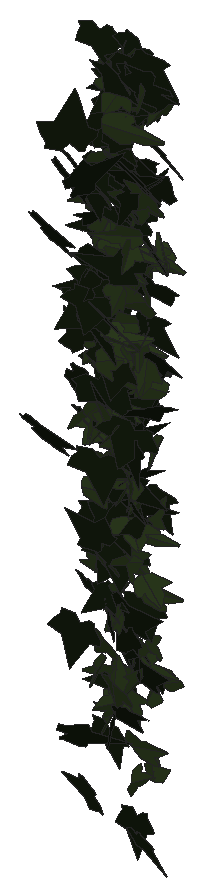
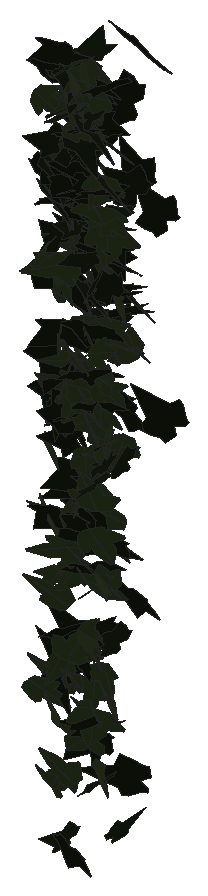
# SketchUp Ruby script. Lengths in millimetres.
U = 1.mm
M = Sketchup.active_model
def pt(a) = Geom::Point3d.new(a.map { |v| v * U })
def face(e, loops, mat)
  f = e.add_face(loops[0].map { |a| pt(a) })
  loops[1..].each { |l| e.add_face(l.map { |a| pt(a) }).erase! }
  f.material = f.back_material = mat if mat
  f
end
# faces: each face lists its corners as indices into pts; further lists are holes
def faces(e, pts, list, mat = nil) = list.each { |f| face(e, (f[0].is_a?(Array) ? f : [f]).map { |l| l.map { |i| pts[i] } }, mat) }
# xy, xz, yz: faces in a plane at the given z, y or x. An outline is a flat list of corners, or four numbers for a rectangle; further outlines are holes
def ring(l) = l.size == 4 ? [[l[0], l[1]], [l[2], l[1]], [l[2], l[3]], [l[0], l[3]]] : l.each_slice(2).to_a
def flat(e, list, mat, &to3) = list.each { |f| face(e, (f[0].is_a?(Array) ? f : [f]).map { |l| ring(l).map { |u, v| to3.(u, v) } }, mat) }
def xy(e, z, list, mat = nil) = flat(e, list, mat) { |x, y| [x, y, z] }
def xz(e, y, list, mat = nil) = flat(e, list, mat) { |x, z| [x, y, z] }
def yz(e, x, list, mat = nil) = flat(e, list, mat) { |y, z| [x, y, z] }
def lines(e, pts, list) = list.each { |a, b| e.add_line(pt(pts[a]), pt(pts[b])) }
# prism: a flat outline (further loops are holes) pulled along v
def prism(e, loops, v, mat = nil)
  f = face(e, loops, mat); d = Geom::Vector3d.new(v.map { |x| x * U })
  f.pushpull(f.normal.samedirection?(d) ? d.length : -d.length)
end
def box(e, o, s, mat = nil) = prism(e, [[o, [o[0] + s[0], o[1], o[2]], [o[0] + s[0], o[1] + s[1], o[2]], [o[0], o[1] + s[1], o[2]]]], [0, 0, s[2]], mat)
def at(x, y, z, deg = 0) = Geom::Transformation.translation(pt([x, y, z])) * Geom::Transformation.rotation(ORIGIN, Z_AXIS, deg.degrees)
def axes(o, x, y, z) = Geom::Transformation.new([*x, 0, *y, 0, *z, 0, *pt(o).to_a, 1])
def part(name) = M.definitions.add(name)
# library, detail: a bought-in or finely detailed component or shape, given as its bounding box
def library(name, o, s) = part(name).tap { |d| box(d.entities, o, s) }
def detail(e, o, s) = box(e.add_group.entities, o, s)
def put(e, d, t, mat = nil) = e.add_instance(d, t).tap { |i| i.material = mat if mat }
def group(e, t, mat = nil) = e.add_group.tap { |g| g.transformation = t; g.material = mat if mat }.entities
root = M.entities
M.materials.add("efeu1").color = [18, 25, 13]
M.materials.add("efeu2").color = [43, 57, 29]
c1 = part("ivyleaf_9")
p = [[39.1,54.8,31.7],[34.5,51.8,30.2],[-5.3,25.2,17.3],[-17.9,28.3,20.9],[-21.6,21.7,17],[-20.2,4.3,5.3],
  [-22.9,-0.3,2.5],[-17.1,-4,-0.6],[-2,-2.1,-1.2],[-0.7,-15.4,-10.1],[16.6,-22.3,-16.7],[21.1,-15.1,-12.5],
  [32.7,-10.7,-11],[46.1,-1.8,-6.6],[30.8,11.2,3.8]]
faces(c1.entities,p,[[0,1,2,3,4,5,6,7,8,9,10,11,12,13,14]],"efeu1")
c2 = part("ivyleaf_10")
p = [[0,12.8,-0.8],[-1.5,51.3,-10.9],[-4.9,51,-11.6],[-13.6,26.5,-7.3],[-13.2,15.9,-4.6],[-21.1,19.3,-7.2],
  [-29.5,16.3,-8.3],[-29.2,8.3,-6.2],[-19.7,-9.8,0.5],[-7.6,-13,4],[1,-12.2,5.8],[-0.4,51.1,-11.1],
  [-1.5,51.1,-10.9],[1,-12.4,5.9],[16.9,-12.4,3.5],[35.1,9.1,-5.1],[35,12.9,-6.1],[20.5,16.4,-4.9],
  [15.8,15,-3.8],[15.3,27.6,-7.1],[12.8,31.3,-7.8]]
faces(c2.entities,p,[[0,1,2,3,4,5,6,7,8,9,10],[11,12,0,13,14,15,16,17,18,19,20]],"efeu2")
put(root,c1,axes([2484.9,735.8,1568],[-1.69227,0.67387,-0.10406],[-0.16332,0.05905,1.11567],[1.2874,0.89329,0.00475]))
put(root,c1,axes([2483.9,756.8,1476.8],[0.18465,0.07319,1.16134],[1.50191,0.8523,-0.11964],[-1.62756,0.7948,0.02135]))
put(root,c1,axes([2359.6,808.1,967.1],[1.40617,-0.08875,-0.62221],[1.17808,-0.06371,0.74411],[-0.20734,-0.96384,0.00811]))
put(root,c1,axes([2446.9,808.4,638.2],[-1.43808,0.002,-0.59826],[1.13852,-0.01008,-0.75558],[-0.01488,-0.96372,0.00666]))
put(root,c1,axes([2369,814.9,1335.4],[1.32826,-0.24708,-0.62973],[1.18689,-0.11557,0.73649],[-0.49882,-0.93289,0.07555]))
put(root,c1,axes([2392.2,851.2,1410.2],[-0.15635,-0.25819,0.96773],[0.53476,-0.93793,-0.22639],[1.82966,0.25207,0.14886]))
put(root,c2,axes([2459.1,851.1,1104.8],[0.566,-0.46163,-0.60165],[0.85277,-0.41442,0.53946],[-1.1644,-0.5279,0.10262]))
put(root,c1,axes([2459.1,853.3,1185.9],[0.68758,-0.5464,0.48417],[0.54213,-0.39189,-0.65481],[1.2793,0.45974,0.01727]))
put(root,c2,axes([2516,854.7,1330],[0.21144,0.59983,-0.55383],[-0.20997,-0.54278,-0.60999],[-1.53954,0.15641,0.00713]))
put(root,c1,axes([2517.1,853.1,1286.2],[-0.55429,0.00633,0.77085],[-1.46054,-0.08043,-0.28928],[0.13896,-0.8201,0.03432]))
put(root,c2,axes([2516.4,856.2,1350.7],[0.02984,0.15758,-0.80777],[-1.38592,-0.37377,-0.08705],[-0.72979,0.71626,0.13228]))
put(root,c1,axes([2435.9,859.7,1206.7],[-0.72098,-0.71589,0.04601],[-0.02643,-0.0447,-0.80989],[1.36503,-0.37898,0.00862]))
put(root,c1,axes([2446.5,861.6,915.6],[-0.48339,-0.87749,-0.09441],[0.07234,0.08727,-0.91342],[1.67811,-0.25653,0.01218]))
put(root,c1,axes([2479.8,871.4,1613.7],[-0.83606,-0.37476,0.71593],[0.0898,-0.82538,-0.4031],[1.53532,-0.1558,0.41343]))
put(root,c1,axes([2425.7,874.3,1149.4],[0.21537,-0.82051,0.52307],[0.37692,-0.49615,-0.82113],[1.81316,0.2006,0.10856]))
put(root,c1,axes([2423.3,881.9,1175.4],[-1.04304,-0.56212,0.5967],[-0.62623,-0.50657,-0.77943],[1.429,-0.63229,0.09397]))
put(root,c1,axes([2441.7,866,1263.9],[-0.16971,-0.08834,0.95115],[1.68448,-0.367,0.04889],[0.68391,0.88201,0.11561]))
put(root,c2,axes([2476.4,871.2,1226.7],[1.15926,-0.71971,0.06776],[0.0676,-0.05871,-0.94281],[1.37415,0.61005,-0.01078]))
put(root,c1,axes([2458.8,884.7,1092.2],[-0.36321,-0.88951,0.3733],[-0.07063,-0.37348,-0.90892],[1.83459,-0.19048,0.03891]))
put(root,c2,axes([2512.3,857.3,886],[0.46586,-0.6296,-0.63071],[-0.12077,0.64009,-0.6636],[1.69178,0.21907,0.1263]))
put(root,c1,axes([2498.5,877.7,947.7],[-0.56617,-0.01021,-0.78546],[1.44293,-0.22351,-0.28423],[-0.3912,-0.80962,0.08837]))
put(root,c1,axes([2500.2,874.9,1413.2],[-1.0248,0.23639,-0.57178],[0.98332,-0.24522,-0.58794],[-0.64782,-0.74615,0.01208]))
put(root,c1,axes([2426.6,863.2,1221.4],[-0.90472,0.61769,0.22037],[-0.29716,0.15775,-0.77898],[-1.21228,-0.49965,0.02649]))
put(root,c2,axes([2474,872,1598.9],[1.5296,-0.57535,-0.12169],[-0.18897,0.07036,-0.98841],[1.10316,0.80981,-0.00058]))
put(root,c2,axes([2460.8,886,955.1],[-0.09591,0.01155,-0.83258],[-0.30336,-0.81881,-0.00171],[-1.55541,0.15899,0.05167]))
put(root,c1,axes([2413.1,859.6,1125.8],[-1.12518,0.24381,-0.4919],[-0.86458,0.18867,0.6395],[0.58672,0.74558,-0.00097]))
put(root,c2,axes([2528.3,868.9,1425.2],[-1.31885,0.28336,0.34939],[-0.66883,0.05958,-0.74533],[-0.53448,-0.77377,0.07056]))
put(root,c1,axes([2494.9,887.1,972.8],[-1.09181,-0.65305,-0.05444],[0.06639,0.04182,-0.86924],[1.24544,-0.57473,-0.00139]))
put(root,c1,axes([2367,892.6,1416.7],[0.54315,-0.58014,0.71659],[0.59216,-0.64553,-0.64653],[1.6518,0.42218,-0.00386]))
put(root,c2,axes([2473.7,889,1111.7],[-0.98102,-0.38488,-0.46913],[-0.56714,-0.37564,0.63561],[-1.00603,0.58709,0.09914]))
put(root,c2,axes([2451.3,880.8,1278.5],[0.56832,0.02888,0.8239],[1.55948,0.08607,-0.3],[-0.17272,0.87211,0.00232]))
put(root,c2,axes([2462,881,1521.9],[0.05458,0.00345,-0.99141],[1.85453,-0.18293,0.02755],[-0.34783,-0.97481,-0.00868]))
put(root,c1,axes([2436.7,872.7,758.5],[-0.24148,0.29665,0.76444],[-0.81568,0.63548,-0.31774],[-1.33046,-0.44344,0.05606]))
put(root,c1,axes([2468.9,881.4,1458.6],[1.70609,-0.3728,-0.19959],[-0.33754,0.09323,-0.9707],[0.7306,0.91364,0.01761]))
put(root,c1,axes([2410.1,903.2,1216],[-0.7247,-0.68788,0.31013],[-0.28527,-0.27151,-0.78624],[1.40746,-0.40922,0.00033]))
put(root,c2,axes([2461.6,874.1,1131.4],[0.41055,-0.12873,-0.94919],[1.27533,0.71553,0.05525],[1.30268,-0.65993,0.24506]))
put(root,c2,axes([2460.8,883.8,494],[-1.27268,0.45432,0.25237],[-0.41429,0.12859,-0.80829],[-0.89816,-0.70308,0.01524]))
put(root,c2,axes([2448,888.4,1286.8],[-0.02144,-0.10949,-0.99075],[1.88284,0.11993,-0.0245],[0.23197,-0.98353,0.10731]))
put(root,c2,axes([2504.1,891.7,1592.1],[0.71636,-0.77323,-0.24016],[-0.08204,0.24533,-0.85743],[1.53877,0.37305,0.06609]))
put(root,c2,axes([2495.2,891.7,1393.8],[-1.7657,-0.00435,0.0386],[-0.07344,-0.00217,-0.92776],[0.00844,-0.92856,0.00198]))
put(root,c1,axes([2491.6,905,524.7],[0.03789,-0.07783,0.86073],[0.75048,-0.7653,-0.07832],[1.46364,0.39442,0.01787]))
put(root,c1,axes([2363.8,901.8,1027],[0.26318,-0.14266,-0.76129],[1.4741,0.02489,0.13602],[-0.0011,-0.77334,0.14481]))
put(root,c2,axes([2419.3,898.7,982.5],[-0.75661,0.59175,-0.36069],[0.35139,-0.31035,-0.71267],[-1.27126,-0.43797,0.01768]))
put(root,c1,axes([2388.7,910.9,1370.4],[-0.02988,-0.7081,0.43658],[0.21345,-0.43447,-0.70065],[1.56876,0.04563,0.10365]))
put(root,c2,axes([2477.4,894.2,1110.8],[-0.623,0.73544,-0.06457],[-0.11512,0.04367,0.80413],[1.40035,0.33078,0.03738]))
put(root,c2,axes([2477.1,896.1,874.1],[0.84548,-0.00115,-0.6705],[-1.2603,0.12545,-0.43895],[0.20023,0.79447,0.06834]))
put(root,c2,axes([2495.8,906.5,519.9],[-0.03194,-0.71517,0.4305],[-0.03508,-0.43017,-0.71533],[1.5883,-0.02388,-0.00714]))
put(root,c1,axes([2474.9,892.2,1506.5],[-1.21577,0.56264,0.37307],[-0.55706,0.232,-0.85107],[-1.15779,-0.70244,0.01773]))
put(root,c2,axes([2415.7,905.7,1131.7],[1.16675,-0.31717,0.59025],[1.00601,-0.26275,-0.6902],[0.78375,0.80943,0.00724]))
put(root,c1,axes([2485.1,909.1,1591.8],[-1.79302,-0.33008,0.09395],[-0.16024,-0.04378,-0.99817],[0.6332,-0.94577,0.01342]))
put(root,c2,axes([2429.3,899.2,689.7],[-1.35531,0.22483,-0.27772],[-0.5332,0.03304,0.74513],[0.42209,0.76365,0.04953]))
put(root,c1,axes([2515.8,904.9,1606.6],[-0.02814,-0.04533,-0.99131],[-1.33466,-0.70098,0.04252],[-1.33625,0.7011,-0.02159]))
put(root,c1,axes([2420,895.8,1034.6],[-0.23842,-0.55746,-0.72596],[0.40486,0.69493,-0.57034],[1.69431,-0.2445,0.03413]))
put(root,c1,axes([2393.2,909.2,261],[0.29829,-0.79501,0.05984],[0.00837,0.06185,0.81015],[-1.51732,-0.15595,0.01623]))
put(root,c2,axes([2459.4,898.9,915.3],[-0.59112,-0.84992,-0.15469],[0.09705,0.14606,-0.90489],[1.64127,-0.31474,-0.0022]))
put(root,c1,axes([2489,907.4,220.9],[0.68986,-0.66754,0.13765],[0.11779,-0.12302,-0.75959],[1.29183,0.3677,-0.00425]))
put(root,c2,axes([2455.9,916.3,1324.7],[-0.34755,0.1429,-0.82601],[0.4308,-0.80557,-0.18941],[-1.53615,-0.25825,0.13376]))
put(root,c2,axes([2505.1,906.1,1219.3],[-0.87736,0.62911,0.2138],[0.24356,-0.17128,0.77993],[1.24089,0.47842,-0.00192]))
put(root,c2,axes([2414.7,919.7,954.5],[0.06673,-0.54942,0.77103],[0.31553,-0.75608,-0.54631],[1.77404,0.15514,0.06816]))
put(root,c2,axes([2500.7,900.3,1204.7],[-0.93079,0.03641,0.64444],[-1.22526,0.03067,-0.49031],[-0.0884,-0.80842,0.01042]))
put(root,c2,axes([2463.4,912.3,1148.3],[0.10461,0.09973,-0.81363],[-1.38113,-0.37331,-0.09478],[-0.72552,0.72503,0.06312]))
put(root,c2,axes([2475.2,902.3,789.6],[1.26142,0.41634,0.17648],[0.27626,0.10067,-0.78267],[-0.81508,0.67845,0.00784]))
put(root,c2,axes([2409.9,909.3,510.2],[0.56971,-0.80877,0.14102],[0.08815,-0.13323,-0.86239],[1.55999,0.30289,-0.00277]))
put(root,c2,axes([2457.7,914.3,707.2],[0.50814,-0.50082,-0.66025],[0.71823,-0.54409,0.56532],[-1.40416,-0.45954,0.05023]))
put(root,c1,axes([2473.9,908.8,801.7],[-1.67884,0.19549,-0.12307],[0.22811,-0.02797,-0.90351],[-0.37584,-0.89022,0.00136]))
put(root,c2,axes([2395.9,905.5,826.4],[0.26841,-0.11162,-0.76977],[1.43793,-0.16626,0.16253],[-0.3518,-0.76471,0.07702]))
put(root,c1,axes([2418.1,902.7,1412.7],[-0.11458,-0.71576,-0.66616],[0.21359,0.65795,-0.71709],[1.84865,-0.12038,0.04156]))
put(root,c1,axes([2426.2,916.4,387.2],[0.16512,0.29022,0.86965],[-0.45978,-0.83543,0.3029],[1.68319,-0.25667,-0.00257]))
put(root,c1,axes([2429.8,922.6,1528.4],[0.02318,-0.06148,-0.96523],[0.50432,-0.92816,0.06246],[-1.77032,-0.26521,0.00516]))
put(root,c2,axes([2409.9,908.9,947.8],[1.16959,0.40623,-0.30525],[-0.49104,-0.16322,-0.73665],[-0.83314,0.66648,0.00565]))
put(root,c1,axes([2357.9,896.6,367.3],[0.86201,0.05067,0.6925],[1.30331,0.10406,-0.45551],[-0.21842,0.82089,0.01499]))
put(root,c2,axes([2432,922.4,442.3],[-0.01005,0.14021,0.91001],[0.20894,-0.90344,0.13984],[1.73987,0.1093,-0.01154]))
put(root,c2,axes([2399.1,917.7,958.5],[0.16243,-0.6148,0.53097],[0.32302,-0.50862,-0.61619],[1.51194,0.17471,0.0746]))
put(root,c2,axes([2384.2,898.3,964.1],[-0.34505,-0.7313,-0.51435],[0.42117,0.47178,-0.74879],[1.64864,-0.27358,0.08364]))
put(root,c2,axes([2375.9,892.5,1130],[-0.17168,-0.51212,0.82096],[0.26811,0.80878,0.52001],[-1.82191,0.16728,-0.00083]))
put(root,c1,axes([2457.5,899.5,861.3],[0.01689,-0.15204,-0.78653],[0.52551,0.73896,-0.13973],[1.43121,-0.26954,0.06059]))
put(root,c2,axes([2390.3,910.2,1229],[0.3966,-0.7691,-0.01612],[-0.00058,0.01662,-0.79682],[1.46408,0.20835,0.00405]))
put(root,c1,axes([2422.3,905.9,1498.2],[0.3294,-0.67643,-0.52752],[-0.12616,0.52599,-0.69622],[1.6277,0.17766,0.05279]))
put(root,c1,axes([2439.9,918.8,732.1],[-0.74317,-0.86408,-0.18766],[0.1456,0.17136,-0.94821],[1.67654,-0.39791,-0.00084]))
put(root,c1,axes([2509.7,896.6,1012.8],[0.80838,0.68591,0.09505],[0.09665,0.08035,-0.80678],[-1.31435,0.42777,-0.00087]))
put(root,c2,axes([2490.5,895,330.6],[-0.08441,-0.2532,-0.78851],[0.39787,0.76065,-0.25601],[1.52512,-0.21245,0.02315]))
put(root,c1,axes([2419.1,923.9,581.6],[-0.08461,0.00443,0.82284],[-0.23626,-0.81465,-0.00232],[1.54814,-0.12408,0.04462]))
put(root,c2,axes([2460.7,901.9,987],[0.37576,0.68911,0.3655],[0.20082,0.34997,-0.71682],[-1.47093,0.22382,-0.0045]))
put(root,c2,axes([2507.7,905.2,694.4],[0.58066,0.71883,0.224],[0.1788,0.20346,-0.78087],[-1.42176,0.31916,-0.00672]))
put(root,c2,axes([2463.8,907.2,1298.9],[0.55177,-0.90055,0.27936],[-0.16476,0.26561,0.94607],[-1.78692,-0.30256,-0.00097]))
put(root,c2,axes([2411,922.7,723.4],[0.44251,-0.75546,0.49666],[0.32069,-0.46763,-0.79018],[1.69053,0.28646,0.01989]))
put(root,c1,axes([2491.5,926.1,1300.7],[0.3191,-0.62273,0.60556],[0.29903,-0.58482,-0.6449],[1.62588,0.22978,-0.00024]))
put(root,c2,axes([2492.2,916.5,1079.2],[1.51671,-0.40304,0.19952],[0.32967,-0.09954,-0.89299],[0.78987,0.81547,-0.0104]))
put(root,c1,axes([2476.7,911.5,1637.2],[-0.28975,-0.36617,-0.83759],[1.2348,0.55489,-0.36051],[1.22559,-0.64562,0.1652]))
put(root,c1,axes([2415.7,931.5,706.6],[-0.365,-0.75154,0.58031],[-0.29867,-0.5588,-0.77555],[1.78226,-0.24756,-0.01112]))
put(root,c1,axes([2454.8,920.6,571.7],[-0.59754,0.07614,-0.87026],[1.6259,-0.16647,-0.32277],[-0.3474,-0.91006,-0.01376]))
put(root,c1,axes([2498.4,909.4,1347.5],[-1.08381,0.40005,0.5151],[-0.86384,0.24796,-0.69438],[-0.89136,-0.72673,0.04663]))
put(root,c1,axes([2414.7,928,632.9],[0.1509,-0.18932,-0.73874],[0.40478,-0.70776,0.20421],[-1.39382,-0.22604,-0.02068]))
put(root,c1,axes([2421.2,915,789.8],[-0.83272,-0.4306,-0.66005],[0.86062,0.48113,-0.61363],[1.2284,-0.62898,-0.01753]))
put(root,c2,axes([2446.7,928,1081],[0.32007,0.25385,-0.85963],[-0.98082,-0.68821,-0.30405],[-1.39572,0.54185,0.01654]))
put(root,c1,axes([2486.8,911.9,1424.9],[0.50363,0.55929,-0.58872],[-0.69098,-0.47236,-0.61194],[-1.38238,0.43987,0.0914]))
put(root,c2,axes([2408.3,923.4,1307.7],[-0.08665,-0.77495,0.37342],[0.17963,-0.37618,-0.76918],[1.6273,0.00026,0.10479]))
put(root,c2,axes([2408.3,920.2,1174.6],[-0.84553,-0.33049,0.57072],[-0.85009,-0.35551,-0.55356],[0.92347,-0.62985,0.01298]))
put(root,c2,axes([2508.8,925.1,1039.5],[0.21911,0.14111,0.83023],[-0.97357,-0.65393,0.18208],[1.27319,-0.52432,-0.00365]))
put(root,c1,axes([2419.3,922.5,843],[0.14826,0.00901,-0.93338],[1.77187,-0.06824,0.07704],[-0.12802,-0.93414,-0.01463]))
put(root,c1,axes([2363.7,920.1,946.5],[0.93276,-0.63824,0.10982],[0.10766,-0.095,-0.80461],[1.22784,0.49319,-0.01287]))
put(root,c2,axes([2466,903.3,853.6],[-0.01823,-0.59114,-0.69461],[0.05802,0.69405,-0.59109],[1.73494,-0.02942,0.01247]))
put(root,c1,axes([2446.3,926.9,1396.9],[0.11451,-0.78991,0.12088],[0.03643,-0.11977,-0.79214],[1.52042,0.06236,0.00987]))
put(root,c2,axes([2495,924.8,1252.1],[0.05538,-0.80641,0.29743],[0.0463,-0.2967,-0.80683],[1.63516,0.03571,0.01277]))
put(root,c1,axes([2444.9,925.3,598.6],[-0.05958,0.01978,0.9289],[1.01582,-0.76038,0.03418],[1.44738,0.53447,0.01425]))
put(root,c1,axes([2510,916.2,1235.1],[0.43999,0.32532,-0.72399],[-1.10177,-0.44678,-0.38561],[-1.03345,0.61481,0.10287]))
put(root,c2,axes([2415.7,920.7,1313.4],[1.4361,-0.16498,0.20367],[0.38222,-0.03491,-0.77235],[0.32054,0.78079,0.00851]))
put(root,c1,axes([2448.2,926.5,1343.7],[0.56205,-0.75516,0.18422],[0.19421,-0.1577,-0.81003],[1.46657,0.31029,0.03666]))
put(root,c1,axes([2413,914.8,1327.2],[0.38222,0.62114,-0.45863],[-0.44727,-0.40223,-0.64766],[-1.39976,0.29813,0.08172]))
put(root,c2,axes([2416,910.7,550],[-1.05159,0.30245,0.48443],[-0.8221,0.2196,-0.62979],[-0.71099,-0.70125,0.01171]))
put(root,c2,axes([2464.7,911.1,719.3],[-0.8336,-0.585,-0.51962],[0.61955,0.40526,-0.73066],[1.35416,-0.54553,0.01442]))
put(root,c1,axes([2475.5,902.3,872.6],[0.58547,0.38852,0.64373],[0.74065,0.51285,-0.4955],[-1.22442,0.496,0.00809]))
put(root,c2,axes([2482.9,921.9,1234.6],[-0.4402,-0.76503,0.07082],[-0.04253,-0.06722,-0.79923],[1.46161,-0.23236,-0.00193]))
put(root,c1,axes([2456.6,918.8,1236.5],[-1.00263,0.57154,-0.16378],[0.20971,-0.12118,-0.7773],[-1.11194,-0.53821,0.00109]))
put(root,c2,axes([2471.1,935.2,820.1],[-0.01269,-0.06635,0.80524],[0.49324,-0.7629,-0.06072],[1.45648,0.25778,0.02758]))
put(root,c2,axes([2467,929.5,1113],[1.24674,-0.50287,0.45753],[0.6897,-0.27931,-0.82584],[1.09478,0.74863,-0.00077]))
put(root,c1,axes([2430.8,912.7,433.1],[1.44082,0.24599,-0.0584],[-0.10558,-0.01826,-0.79601],[-0.46945,0.75908,-0.00022]))
put(root,c1,axes([2446.1,915,775.9],[-1.27399,-0.04287,0.56254],[1.0704,0.01804,0.67062],[-0.08457,0.87419,0.01375]))
put(root,c2,axes([2477.6,929,518],[0.25226,-0.19964,-0.90011],[1.49313,-0.45326,0.21606],[-0.92174,-0.78888,0.10365]))
put(root,c1,axes([2476.8,907.9,942.6],[0.23293,0.16249,0.78214],[1.04208,0.5591,-0.20183],[-1.10704,0.56047,-0.02542]))
put(root,c2,axes([2465.3,939.9,536.6],[-0.11754,0.05224,0.89195],[0.76689,-0.79637,0.07454],[1.51773,0.40644,0.03141]))
put(root,c2,axes([2433.1,923.7,598.5],[0.89259,-0.61779,-0.19979],[-0.22972,0.15921,-0.77564],[1.21419,0.48428,0.00012]))
put(root,c2,axes([2471.7,925,1053.7],[1.17141,-0.75122,-0.17987],[-0.2126,0.14101,-0.97116],[1.45468,0.62554,0.00291]))
put(root,c1,axes([2510.7,909.6,1418.1],[-0.06632,0.7785,0.36985],[0.00279,0.3702,-0.77911],[-1.64035,-0.03085,-0.01628]))
put(root,c1,axes([2414.7,943.9,1245.3],[-0.12442,-0.32194,0.83628],[-0.37562,-0.81274,-0.32831],[1.66359,-0.20758,-0.01158]))
put(root,c1,axes([2377.2,940,1253.4],[0.16331,-0.37368,0.77978],[0.4578,-0.74237,-0.38222],[1.58073,0.25361,0.03013]))
put(root,c2,axes([2398.1,934.3,1070.8],[-0.59087,-0.5235,0.43837],[-0.36605,-0.39501,-0.60793],[1.24689,-0.36404,0.02926]))
put(root,c2,axes([2438.6,925.1,1566.7],[-1.27433,0.04161,-0.52033],[0.98633,-0.04814,-0.67075],[-0.11871,-0.84661,0.01257]))
put(root,c1,axes([2365.1,936.8,629.1],[0.66777,-0.69906,0.30878],[0.25994,-0.27694,-0.78217],[1.43104,0.37651,-0.00201]))
put(root,c2,axes([2487.7,927.9,658.8],[-0.65021,-0.02507,0.77516],[1.46605,0.08746,0.34233],[-0.17153,0.84258,-0.01247]))
put(root,c1,axes([2488.7,935.6,1482.5],[0.77329,-0.63201,0.30507],[0.30951,-0.25812,-0.75135],[1.29929,0.43764,-0.00258]))
put(root,c2,axes([2427.5,937.7,1167.9],[0.73963,-0.53363,0.52554],[0.69245,-0.38302,-0.65795],[1.24595,0.52964,0.05369]))
put(root,c2,axes([2505.7,935.1,933.8],[0.7025,-0.7897,0.23296],[0.19973,-0.20809,-0.87168],[1.55421,0.38369,0.00672]))
put(root,c2,axes([2518.3,940.1,1558.4],[-0.22165,-0.64906,0.53325],[0.0065,-0.53871,-0.65496],[1.5987,-0.0878,0.07659]))
put(root,c2,axes([2435,925.6,1631],[-0.07047,-0.83015,-0.259],[-0.00316,0.2593,-0.83088],[1.65504,-0.03485,-0.01261]))
put(root,c1,axes([2523.2,918.7,1399.3],[0.11017,-0.03016,0.91369],[-0.78554,0.81603,0.05309],[-1.55245,-0.41505,0.03798]))
put(root,c2,axes([2450.6,941.5,1620.6],[0.32397,-0.68568,0.54442],[0.37514,-0.51036,-0.70442],[1.62353,0.25475,0.05413]))
put(root,c1,axes([2434.4,935.1,1305.8],[-1.28333,0.00539,0.4409],[-0.83907,0.00467,-0.67432],[-0.01345,-0.80564,-0.00096]))
put(root,c1,axes([2473,947.8,1549.7],[-0.61076,-0.52157,0.60758],[-0.26488,-0.60827,-0.59566],[1.50078,-0.31961,0.14213]))
put(root,c1,axes([2457.6,936.6,1501.8],[-1.10585,0.36774,-0.43299],[0.50293,-0.37331,-0.67167],[-0.95707,-0.62108,0.14734]))
put(root,c2,axes([2406.4,924.8,1434.4],[-0.78372,-0.65559,-0.37988],[0.39015,0.31983,-0.77419],[1.38827,-0.45999,0.00312]))
put(root,c2,axes([2408.1,933.3,1589.8],[-0.44047,0.00481,-0.83159],[1.5165,-0.24578,-0.22318],[-0.453,-0.82746,0.06145]))
put(root,c1,axes([2391.3,949.3,934.2],[-0.42524,-0.26499,0.81358],[-0.2734,-0.81731,-0.30565],[1.60535,-0.20938,0.16345]))
put(root,c2,axes([2391,929.8,1349.7],[-1.14322,-0.74217,-0.1277],[0.15629,0.09782,-0.95479],[1.4247,-0.60627,0.00227]))
put(root,c2,axes([2384.3,940,1088],[-0.07312,-0.19654,0.74734],[1.33859,-0.31884,-0.0477],[0.6092,0.677,0.1945]))
put(root,c1,axes([2435.6,932.9,801],[0.38421,-0.06845,0.80448],[1.41105,-0.3126,-0.21265],[0.60837,0.76826,-0.01485]))
put(root,c1,axes([2455,946.2,1005.6],[-0.5463,-0.84979,0.06163],[-0.02888,-0.05993,-0.89694],[1.6213,-0.2874,0.00479]))
put(root,c2,axes([2391.8,932.3,1380.5],[-1.4389,0.05552,-0.23432],[0.43591,-0.07256,-0.75621],[-0.14149,-0.78819,0.05311]))
put(root,c1,axes([2467.8,928.2,1149.9],[-0.31222,-0.2719,-0.80747],[0.74742,0.70562,-0.31739],[1.43905,-0.42548,-0.01035]))
put(root,c2,axes([2425.1,930.6,470.6],[1.29086,-0.42746,0.19087],[-0.29936,0.10839,0.80169],[-0.83917,-0.69621,0.00762]))
put(root,c1,axes([2488.7,926.4,1096.7],[1.52897,0.10893,-0.41678],[-0.78579,-0.05692,-0.81072],[-0.23391,0.90325,-0.00082]))
put(root,c2,axes([2414.1,936.3,862.1],[-1.46478,-0.15658,0.27459],[0.53207,0.00012,0.78365],[-0.28076,0.81716,0.0525]))
put(root,c2,axes([2460.5,936.4,1526.4],[-0.23823,0.77309,-0.29128],[0.13421,-0.28353,-0.78283],[-1.56658,-0.14186,-0.02277]))
put(root,c2,axes([2491.9,924.1,1143.4],[0.23183,-0.46759,-0.59193],[-0.07982,0.59447,-0.47823],[1.43343,0.10873,0.0691]))
put(root,c1,axes([2456.3,951.5,1632.5],[-0.51589,-0.63117,0.50294],[-0.14703,-0.50782,-0.67893],[1.52891,-0.26181,0.10441]))
put(root,c2,axes([2455.8,927.8,1100.8],[-0.23472,-0.24858,-0.70562],[1.27183,0.2849,-0.21717],[0.6401,-0.65722,0.17275]))
put(root,c2,axes([2453.6,944.3,581.6],[-0.99077,-0.5539,-0.47104],[-0.61743,-0.34152,0.76013],[-1.23845,0.61339,-0.00213]))
put(root,c2,axes([2404.5,937.4,1389.9],[1.55901,0.21802,-0.21675],[-0.40204,-0.049,-0.84764],[-0.42509,0.84592,0.00676]))
put(root,c1,axes([2451.1,937.2,996.3],[1.2422,0.59618,0.38423],[-0.55544,-0.25016,0.88392],[1.23031,-0.71488,0.01112]))
put(root,c2,axes([2453.9,948.9,1588.7],[0.25835,-0.56849,0.65049],[0.4816,-0.60342,-0.58016],[1.57205,0.27828,0.07083]))
put(root,c1,axes([2397.5,932.1,1423.4],[0.34488,-0.55981,-0.54317],[0.28899,0.57229,-0.53916],[1.45612,0.01901,0.23566]))
put(root,c1,axes([2452.4,935.2,754.6],[-1.47675,0.48403,0.02133],[-0.03444,0.01128,-0.91452],[-0.92146,-0.77614,0.00001]))
put(root,c1,axes([2499.1,927.7,523.1],[0.52719,0.05335,-0.76462],[-1.45461,0.08051,-0.27127],[0.10996,0.80925,0.0774]))
put(root,c2,axes([2493.6,941.1,796.7],[0.86123,-0.70845,-0.29478],[0.29612,-0.2504,0.84063],[-1.43005,-0.47851,-0.00346]))
put(root,c1,axes([2457.2,942.6,230.1],[-1.02801,0.06198,-0.66742],[1.26663,-0.05239,-0.54348],[-0.15177,-0.85701,-0.01504]))
put(root,c1,axes([2468.7,919.2,1590.5],[0.18489,0.69874,0.51085],[0.12921,0.50632,-0.70545],[-1.64226,0.1185,0.00201]))
put(root,c1,axes([2396.3,948.5,367.6],[0.07098,-0.79551,0.19246],[0.01864,-0.19221,-0.79638],[1.55757,0.03855,0.00076]))
put(root,c1,axes([2456.8,953.7,1550.4],[-0.39833,-0.74721,0.42147],[0.05879,-0.44011,-0.76492],[1.63166,-0.16656,0.13045]))
put(root,c1,axes([2419.4,947.3,1097.9],[-0.78501,-0.80289,-0.14445],[0.12743,0.12799,-0.90264],[1.54735,-0.41787,0.00106]))
put(root,c2,axes([2449.8,940.1,1587.4],[0.57764,-0.80065,-0.01801],[-0.007,0.01787,-0.85624],[1.52417,0.30352,0.00289]))
put(root,c1,axes([2405.5,948.2,1046.2],[-0.97401,-0.59635,-0.02477],[0.03738,0.01579,-0.78583],[1.13534,-0.51213,0.00462]))
put(root,c2,axes([2437.9,941,1098.5],[1.01601,-0.47088,-0.34601],[0.55595,-0.19085,0.71041],[-0.96319,-0.60687,0.04506]))
put(root,c1,axes([2453,940,1429.2],[0.32409,0.49004,-0.61455],[-0.31346,-0.5926,-0.51818],[-1.46272,0.23557,-0.02512]))
put(root,c2,axes([2450.2,933.2,1037.1],[-0.92525,-0.59628,-0.33744],[0.42548,0.25305,-0.76925],[1.23258,-0.53495,0.01224]))
put(root,c2,axes([2438.3,952,1533.7],[-0.64783,-0.35279,0.70404],[-0.28272,-0.72446,-0.43484],[1.47183,-0.29444,0.22636]))
put(root,c1,axes([2414.6,943.9,1182],[-1.02767,-0.48823,-0.41615],[0.55754,0.29625,-0.72769],[1.08621,-0.61399,-0.0202]))
put(root,c2,axes([2522.9,926.5,1269.5],[-0.11841,0.74109,-0.54363],[-0.18287,0.53665,0.74256],[1.73965,0.10685,0.04105]))
put(root,c1,axes([2479.1,951.8,1396.8],[-0.60548,-0.73627,0.1545],[-0.14338,-0.13572,-0.80192],[1.42459,-0.32659,-0.01505]))
put(root,c2,axes([2461.3,942.4,357.3],[-0.89419,-0.01352,0.68213],[1.29518,-0.0684,0.46737],[0.09268,0.82545,0.04991]))
put(root,c2,axes([2507.8,948.2,1262.6],[0.15744,0.50797,0.62453],[-0.34848,-0.5995,0.51186],[1.49199,-0.19362,0.05365]))
put(root,c2,axes([2418.4,952.7,632.5],[0.1451,-0.55451,0.6336],[0.14376,-0.62912,-0.55968],[1.596,0.10708,-0.00719]))
put(root,c2,axes([2468,923.2,1071.6],[0.01015,-0.44816,-0.88066],[0.18624,0.87658,-0.4455],[1.87137,-0.08481,0.04911]))
put(root,c2,axes([2394.8,954.6,1144.2],[0.02319,-0.16551,0.77293],[0.18306,-0.76697,-0.16575],[1.49321,0.09659,0.00832]))
put(root,c2,axes([2468,931.4,760.1],[-0.51125,-0.16514,-0.80042],[1.38543,0.33466,-0.31335],[0.70707,-0.77513,0.03523]))
put(root,c1,axes([2400.4,948.2,904.1],[0.40892,-0.80881,0.04294],[0.02615,-0.04078,-0.83686],[1.54128,0.21528,0.0028]))
put(root,c2,axes([2417.8,943.8,1014.7],[0.44737,-0.75198,0.05685],[0.04681,-0.05187,-0.78783],[1.4345,0.23621,0.00798]))
put(root,c1,axes([2501.1,924.7,992.4],[-0.41905,0.18806,-0.79851],[-1.14381,0.52578,0.28954],[1.06272,0.64005,-0.00323]))
put(root,c1,axes([2465.6,949.3,623.1],[-0.23456,-0.77998,-0.09236],[0.03248,0.09081,-0.78966],[1.49448,-0.12439,0.00266]))
put(root,c2,axes([2397.9,945.2,390.7],[0.5366,-0.793,0.06815],[0.05681,-0.06171,-0.8416],[1.51374,0.28342,0.00743]))
put(root,c2,axes([2499.9,936,326.1],[1.06443,-0.32441,0.39513],[-0.63598,0.21125,0.64644],[-0.73638,-0.65138,0.01286]))
put(root,c1,axes([2407.2,944.3,1313.9],[1.14555,-0.66537,-0.00201],[-0.00247,0.00154,-0.89722],[1.26634,0.60191,0.00007]))
put(root,c1,axes([2408.4,950.8,1556.6],[0.56359,-0.74041,0.23584],[0.22319,-0.20691,-0.79684],[1.46197,0.31702,0.03073]))
put(root,c2,axes([2483.4,933.6,556.7],[-0.36307,-0.67734,-0.5132],[0.45815,0.46136,-0.6984],[1.55111,-0.29482,0.08616]))
put(root,c2,axes([2404.5,947.5,810.1],[-0.86551,-0.66197,0.34515],[-0.33296,-0.2984,-0.80281],[1.38127,-0.48673,0.02276]))
put(root,c2,axes([2440.4,941.3,1062.6],[-0.1775,0.00454,-0.8347],[1.57827,-0.09524,-0.09318],[-0.18109,-0.83448,0.00609]))
put(root,c1,axes([2445.4,958.3,1526.8],[-1.10293,-0.41741,0.38754],[-0.42633,-0.34129,-0.70256],[0.99667,-0.6079,0.12833]))
put(root,c2,axes([2440.6,955,1569.7],[0.1006,-0.68254,0.49372],[0.4297,-0.46511,-0.66717],[1.54458,0.17385,0.15345]))
put(root,c2,axes([2411.8,948,1013.9],[1.14466,-0.09468,0.57021],[1.07806,-0.06728,-0.60864],[0.21901,0.82604,0.01579]))
put(root,c1,axes([2426,958,460.1],[-0.51955,-0.1747,0.71214],[-1.06786,-0.43945,-0.32289],[0.89845,-0.62334,0.02804]))
put(root,c2,axes([2477.3,937.1,1269.2],[-0.89094,-0.20873,-0.75076],[1.32622,0.27985,-0.51231],[0.66375,-0.83933,0.01589]))
put(root,c2,axes([2488.7,941.7,460.4],[0.88138,-0.67856,0.1728],[-0.1111,0.16904,0.82023],[-1.32801,-0.46449,0.04606]))
put(root,c1,axes([2374.3,952.9,1633.8],[-0.14019,-0.85929,-0.13451],[0.03032,0.13363,-0.86243],[1.65503,-0.07523,0.00441]))
put(root,c2,axes([2410.3,943.1,482.5],[-1.39199,-0.49272,-0.07491],[0.11819,0.04189,-0.88188],[0.94113,-0.73402,-0.00005]))
put(root,c2,axes([2386.7,948.7,1041.5],[1.35605,-0.28692,0.18707],[0.33789,-0.05987,-0.76804],[0.55747,0.73422,0.01048]))
put(root,c2,axes([2518.1,949.2,503.1],[-0.70692,-0.14663,0.6472],[-1.08251,-0.31172,-0.39705],[0.6506,-0.67799,0.04258]))
put(root,c1,axes([2504.1,932,1381.4],[-0.39508,0.6106,0.49817],[-0.30589,0.47153,-0.64492],[-1.46827,-0.26254,0.00031]))
put(root,c2,axes([2422.2,946.6,440.4],[1.33127,0.06896,0.43914],[0.82919,0.05614,-0.70279],[-0.16791,0.824,0.01113]))
put(root,c1,axes([2434,938.6,1545.4],[-0.75813,0.77075,0.07487],[-0.06048,0.06785,-0.8676],[-1.47256,-0.3996,-0.00291]))
put(root,c1,axes([2397.6,959.1,972.7],[-0.26853,-0.77425,0.21004],[-0.05597,-0.20813,-0.78696],[1.52578,-0.1439,0.0081]))
put(root,c1,axes([2470,947.2,827.1],[-0.60618,-0.40667,-0.6645],[0.90074,0.46923,-0.51401],[1.17775,-0.56818,0.05111]))
put(root,c1,axes([2405.8,944.4,1461.7],[-1.09042,0.562,-0.04025],[0.05325,-0.02896,-0.80256],[-1.07102,-0.57362,0.00108]))
put(root,c1,axes([2441.5,938.7,1511.7],[-0.2378,0.81723,-0.06658],[0.03234,-0.06475,-0.8267],[-1.56018,-0.12591,-0.00699]))
